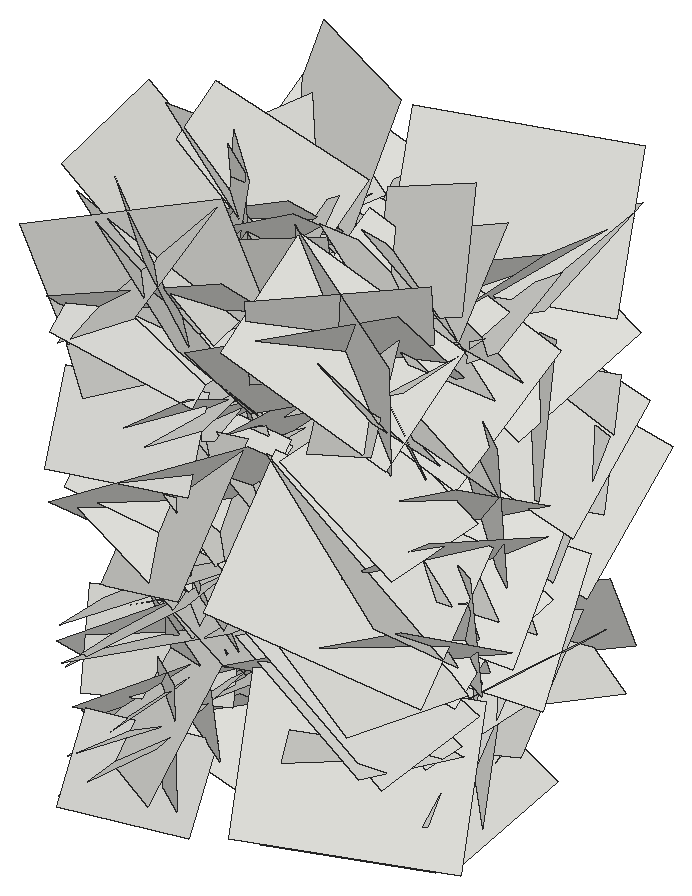
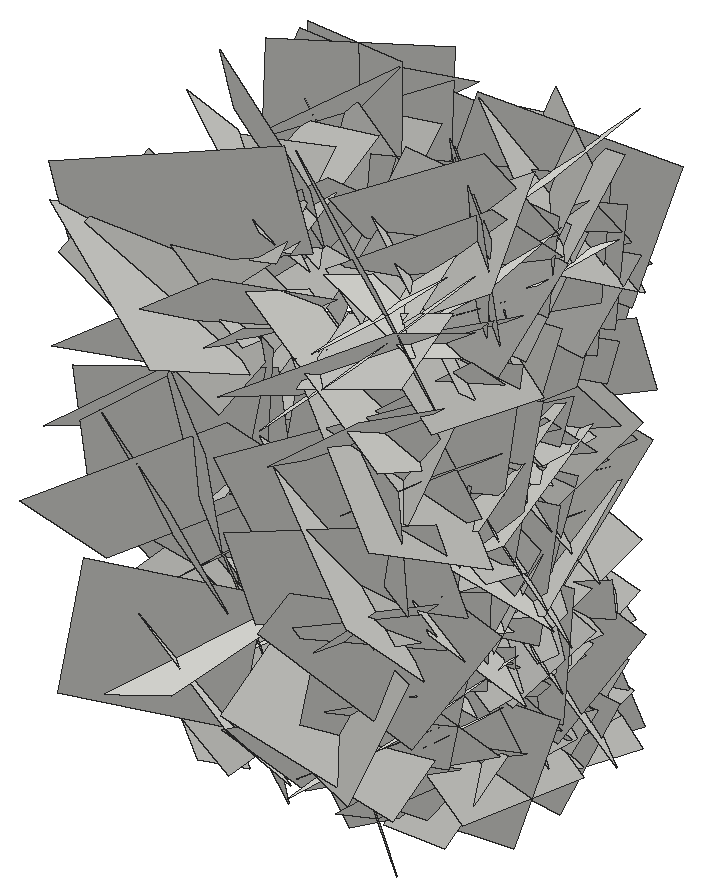
# SketchUp Ruby script. Lengths in inches.
U = 1.inch
M = Sketchup.active_model
def pt(a) = Geom::Point3d.new(a.map { |v| v * U })
def face(e, loops, mat)
  f = e.add_face(loops[0].map { |a| pt(a) })
  loops[1..].each { |l| e.add_face(l.map { |a| pt(a) }).erase! }
  f.material = f.back_material = mat if mat
  f
end
# faces: each face lists its corners as indices into pts; further lists are holes
def faces(e, pts, list, mat = nil) = list.each { |f| face(e, (f[0].is_a?(Array) ? f : [f]).map { |l| l.map { |i| pts[i] } }, mat) }
# xy, xz, yz: faces in a plane at the given z, y or x. An outline is a flat list of corners, or four numbers for a rectangle; further outlines are holes
def ring(l) = l.size == 4 ? [[l[0], l[1]], [l[2], l[1]], [l[2], l[3]], [l[0], l[3]]] : l.each_slice(2).to_a
def flat(e, list, mat, &to3) = list.each { |f| face(e, (f[0].is_a?(Array) ? f : [f]).map { |l| ring(l).map { |u, v| to3.(u, v) } }, mat) }
def xy(e, z, list, mat = nil) = flat(e, list, mat) { |x, y| [x, y, z] }
def xz(e, y, list, mat = nil) = flat(e, list, mat) { |x, z| [x, y, z] }
def yz(e, x, list, mat = nil) = flat(e, list, mat) { |y, z| [x, y, z] }
def lines(e, pts, list) = list.each { |a, b| e.add_line(pt(pts[a]), pt(pts[b])) }
# prism: a flat outline (further loops are holes) pulled along v
def prism(e, loops, v, mat = nil)
  f = face(e, loops, mat); d = Geom::Vector3d.new(v.map { |x| x * U })
  f.pushpull(f.normal.samedirection?(d) ? d.length : -d.length)
end
def box(e, o, s, mat = nil) = prism(e, [[o, [o[0] + s[0], o[1], o[2]], [o[0] + s[0], o[1] + s[1], o[2]], [o[0], o[1] + s[1], o[2]]]], [0, 0, s[2]], mat)
def at(x, y, z, deg = 0) = Geom::Transformation.translation(pt([x, y, z])) * Geom::Transformation.rotation(ORIGIN, Z_AXIS, deg.degrees)
def axes(o, x, y, z) = Geom::Transformation.new([*x, 0, *y, 0, *z, 0, *pt(o).to_a, 1])
def part(name) = M.definitions.add(name)
# library, detail: a bought-in or finely detailed component or shape, given as its bounding box
def library(name, o, s) = part(name).tap { |d| box(d.entities, o, s) }
def detail(e, o, s) = box(e.add_group.entities, o, s)
def put(e, d, t, mat = nil) = e.add_instance(d, t).tap { |i| i.material = mat if mat }
def group(e, t, mat = nil) = e.add_group.tap { |g| g.transformation = t; g.material = mat if mat }.entities
root = M.entities
c1 = part("Component\#6")
p = [[0.01,0,0],[0,3.24,4.54],[4.32,3.24,4.54],[4.33,0,0]]
faces(c1.entities,p,[[0,1,2,3]])
put(root,c1,axes([24.34,188.38,23.95],[-0.14683,-0.05211,-1.06804],[-0.1506,-1.06652,0.07046],[1.12342,-0.14978,-0.13015]))
put(root,c1,axes([28.31,187.95,18.35],[0.24952,-0.85217,0.60628],[0.01294,0.62364,0.87183],[-1.1085,-0.18454,0.14665]))
put(root,c1,axes([28.31,184.68,7.1],[0.07537,-0.21143,-0.85755],[0.01444,-0.85996,0.21315],[-0.93612,-0.03029,-0.06575]))
put(root,c1,axes([24.34,184.16,21.8125],[-0.07155,0.99261,-0.10082],[-0.11355,-0.10768,-0.9884],[1.05147,0.05592,-0.1136]))
put(root,c1,axes([24.34,192.04,5.47],[-0.24252,-0.79203,0.72828],[-0.0092,0.7459,0.80846],[1.14049,-0.1624,0.16139]))
put(root,c1,axes([24.34,189.65,5.54],[0.06955,0.77959,0.08211],[0.00823,0.08175,-0.78235],[0.8309,-0.06607,0.00087]))
put(root,c1,axes([24.34,189.86,21.06],[-0.09411,0.75469,-0.30292],[0.23058,-0.27158,-0.74036],[0.83059,0.16091,0.17121]))
put(root,c1,axes([24.34,184.33,2.33],[-0.23495,-0.78095,0.69461],[0.033,0.70481,0.80235],[1.10738,-0.18669,0.12346]))
put(root,c1,axes([28.31,182.875,15.8],[0.04284,-0.30855,-0.78276],[0.017,-0.78324,0.30957],[-0.8917,-0.02976,-0.0317]))
put(root,c1,axes([28.31,183.91,5.17],[0.1157,0.58195,-0.7538],[0.08085,-0.76164,-0.57696],[-1.0062,0.00571,-0.13304]))
put(root,c1,axes([28.31,180.19,4.07],[-0.08532,0.68038,-0.07405],[-0.04058,-0.07892,-0.68351],[-0.72433,-0.07573,0.04702]))
put(root,c1,axes([28.31,182.98,9.92],[-0.09782,-0.62966,-0.10425],[-0.08997,-0.09229,0.63256],[-0.67052,0.10424,-0.06967]))
put(root,c1,axes([28.31,190.84,12.42],[-0.00848,-0.77925,-0.15089],[0.03038,-0.15108,0.77873],[-0.8408,0.0024,0.02966]))
put(root,c1,axes([28.31,191.35,2.27],[0.06694,-0.86655,-0.10749],[0.04783,-0.10439,0.86806],[-0.92435,-0.06816,0.03713]))
put(root,c1,axes([28.31,191.46,9.82],[0.08538,-0.06629,-0.92063],[0.09555,-0.91915,0.07407],[-0.97372,-0.09601,-0.07345]))
put(root,c1,axes([28.31,193.37,9.31],[0.05697,-0.46717,-0.61186],[-0.09106,-0.61316,0.46062],[-0.81091,0.03603,-0.09471]))
put(root,c1,axes([28.31,183.28,17.73],[0.09647,-0.26045,0.74001],[-0.11879,0.73302,0.27177],[-0.82305,-0.13632,0.04751]))
put(root,c1,axes([28.31,185.14,8.49],[-0.08576,-0.66072,-0.04627],[-0.0456,-0.04128,0.66459],[-0.70059,0.08356,-0.03759]))
put(root,c1,axes([28.31,192.03,8.33],[0.03388,0.22508,-0.86549],[0.13142,-0.8588,-0.21876],[-0.93879,-0.1121,-0.06186]))
put(root,c1,axes([24.34,192.08,20.31],[0.05296,-0.67773,-0.30339],[0.1724,-0.2867,0.66724],[0.76797,0.11109,-0.12886]))
put(root,c1,axes([24.34,184.53,11.29],[-0.10396,-0.95246,0.37472],[-0.04499,0.37989,0.95451],[1.084,-0.07558,0.07555]))
put(root,c1,axes([28.31,183.19,13.8],[0.02762,0.65605,0.3231],[-0.06014,0.32414,-0.6536],[-0.77284,-0.00178,0.06241]))
put(root,c1,axes([28.31,185.94,13.1875],[0.12339,0.16979,-0.82402],[-0.01755,-0.83125,-0.17361],[-0.89164,0.03986,-0.11061]))
put(root,c1,axes([28.31,185.26,12.26],[0.159,0.84642,0.10737],[-0.04855,0.11685,-0.85715],[-0.9031,0.14274,0.06498]))
put(root,c1,axes([24.34,181.6,11.88],[0.05183,0.72565,0.67247],[-0.15864,0.67097,-0.71314],[1.03662,0.0664,-0.14276]))
put(root,c1,axes([28.31,192.38,19.24],[-0.04943,-0.7355,0.057],[0.07325,0.05251,0.73407],[-0.77853,0.05163,0.06545]))
put(root,c1,axes([24.34,185.13,2.21],[0.09174,0.69928,0.36],[0.10121,0.35015,-0.7031],[0.82753,-0.12035,0.04608]))
put(root,c1,axes([24.34,185.25,15.47],[0.04372,0.77316,0.71524],[-0.20224,0.70943,-0.75587],[1.09798,0.09988,-0.16771]))
put(root,c1,axes([24.34,183.61,1.59],[0.06331,-0.78644,0.46242],[-0.03597,0.46118,0.7887],[0.96639,0.06869,-0.00094]))
put(root,c1,axes([24.34,186.63,-0.64],[-0.14781,-0.37723,1.01914],[-0.01271,1.02797,0.37886],[1.15185,-0.03706,0.13496]))
put(root,c1,axes([24.34,183.46,7.83],[-0.1867,0.36795,-0.96583],[0.13041,-0.96532,-0.39019],[1.08777,0.17888,-0.11899]))
put(root,c1,axes([28.31,192.83,7.86],[-0.1126,-0.65912,-0.17655],[0.1088,-0.19208,0.65534],[-0.71507,0.07456,0.12751]))
put(root,c1,axes([28.31,183.375,2.21],[-0.01982,-0.33114,-0.74136],[0.16849,-0.7287,0.32148],[-0.84401,-0.13769,0.08159]))
put(root,c1,axes([24.34,187.85,22.99],[0.09057,-0.06637,-0.91857],[-0.07612,-0.92019,0.05981],[0.97325,-0.06579,0.09016]))
put(root,c1,axes([24.34,187.17,12.95],[-0.05814,-0.16279,1.09674],[-0.14666,1.09051,0.15494],[1.1661,0.12904,0.07417]))
put(root,c1,axes([24.34,185.08,2.16],[0.06404,-1.02262,-0.11109],[-0.17979,-0.11966,1.00929],[1.07543,0.04089,0.17535]))
put(root,c1,axes([24.34,180.14,11.99],[-0.0212,0.75168,0.8023],[-0.17372,0.79143,-0.74558],[1.15236,0.13314,-0.09764]))
put(root,c1,axes([28.31,186.92,8.78],[0.10246,-0.30095,0.75916],[0.04625,0.76527,0.29782],[-0.86439,0.00528,0.10592]))
put(root,c1,axes([24.34,191,16.96],[-0.17643,-1.14926,-0.11809],[-0.05518,-0.11173,1.16072],[1.22339,-0.17078,0.03532]))
put(root,c1,axes([24.34,189.57,16.9],[0.06471,0.53395,-0.71324],[0.01751,-0.71546,-0.53421],[0.94426,-0.02333,0.05878]))
put(root,c1,axes([28.31,184.43,15.42],[0.12844,-0.04329,0.74472],[-0.08874,0.74892,0.05716],[-0.78574,-0.09166,0.11528]))
put(root,c1,axes([24.34,179.97,24.47],[-0.23304,1.36821,0.06434],[-0.25904,0.02493,-1.36533],[1.42861,0.2277,-0.23708]))
put(root,c1,axes([24.34,190.33,17.67],[0.17424,0.82504,0.17436],[-0.04616,0.18571,-0.83769],[0.89267,-0.15144,-0.07735]))
put(root,c1,axes([24.34,186.72,4.72],[-0.08241,-0.91883,0.29273],[0.13826,0.28096,0.91654],[1.0128,-0.11312,-0.1013]))
put(root,c1,axes([24.34,185.64,19.96],[-0.2349,1.07139,0.39402],[0.08081,0.41437,-1.08385],[1.20734,0.18072,0.1492]))
put(root,c1,axes([28.31,184.54,3.47],[0.05739,0.5962,-0.42459],[0.0201,-0.42675,-0.59681],[-0.77559,0.03305,-0.04688]))
put(root,c1,axes([28.31,189.45,1.42],[-0.1039,0.30381,0.53974],[0.07033,0.54846,-0.29667],[-0.65275,0.01074,-0.11787]))
put(root,c1,axes([24.34,186.9375,3.03],[0.11563,0.62873,-0.58509],[0.05581,-0.59358,-0.62803],[0.90867,-0.04354,0.11303]))
put(root,c1,axes([24.34,184.51,1.15],[-0.01173,-1.06899,-0.22188],[-0.10644,-0.21996,1.06472],[1.15237,-0.0312,0.09608]))
put(root,c1,axes([28.31,183.83,7.3125],[0.02805,0.62389,-0.09529],[-0.05665,-0.09282,-0.62253],[-0.66659,0.03414,0.0489]))
put(root,c1,axes([28.31,183.1,18.89],[0.1435,0.17311,-0.85276],[0.14536,-0.85648,-0.1521],[-0.91084,-0.10941,-0.15862]))
put(root,c1,axes([24.34,187.61,11.62],[-0.28203,-0.58282,-1.12773],[0.01249,-1.15332,0.59327],[1.34554,-0.11146,-0.24188]))
put(root,c1,axes([24.34,184.19,13.53],[0.08078,-0.49886,0.79857],[0.01528,0.8017,0.49945],[0.99796,0.02811,-0.07229]))
put(root,c1,axes([24.34,181.29,16.68],[0.08133,-0.245,0.96212],[-0.05676,0.96256,0.24939],[1.05086,0.07095,-0.06099]))
put(root,c1,axes([28.31,186.0625,6.1],[0.08854,0.52684,0.45627],[-0.00383,0.45985,-0.53032],[-0.73876,0.06076,0.05744]))
put(root,c1,axes([28.31,187.98,11.49],[0.12716,0.81746,0.20835],[0.15,0.18797,-0.81896],[-0.88154,0.1499,-0.10929]))
put(root,c1,axes([24.34,194.3,13.93],[-0.22437,-1.23478,-0.60854],[-0.19245,-0.58527,1.25072],[1.44644,-0.26941,0.07201]))
put(root,c1,axes([24.34,184.41,20.14],[-0.03821,-1.03167,-0.60174],[-0.15497,-0.59368,1.0266],[1.25647,-0.1046,0.10832]))
put(root,c1,axes([28.31,186.3,8.38],[-0.07617,0.47932,0.41871],[0.13681,0.42359,-0.46276],[-0.66062,0.03245,-0.14411]))
put(root,c1,axes([24.34,184.31,4.6],[0.1576,-0.1516,-1.0147],[-0.15202,-1.0183,0.13112],[1.07684,-0.12157,0.16702]))
put(root,c1,axes([24.34,179.32,18.3],[0.15069,0.54422,0.74866],[-0.00735,0.75804,-0.54972],[0.98107,-0.07791,-0.11911]))
put(root,c1,axes([28.31,188.8,6.44],[0.14743,-0.18272,-0.74199],[0.06403,-0.74919,0.19581],[-0.80747,-0.09277,-0.11994]))
put(root,c1,axes([24.34,185.52,6.2],[-0.2751,-0.65276,-1.16933],[-0.03559,-1.18754,0.67037],[1.41909,-0.15632,-0.20987]))
put(root,c1,axes([24.34,181.08,20.02],[-0.00536,1.00575,0.03656],[0.10796,0.03689,-1.00058],[1.06133,0.00133,0.10197]))
put(root,c1,axes([24.34,184.05,20.67],[0.10102,0.73684,0.6989],[-0.04073,0.70408,-0.73707],[1.07574,-0.04254,-0.09354]))
put(root,c1,axes([24.34,191.125,9.45],[-0.23474,-0.88576,-0.93612],[0.00151,-0.95001,0.89856],[1.36608,-0.15116,-0.16185]))
put(root,c1,axes([24.34,185.11,13.22],[0.08906,-0.95701,-0.12674],[0.0585,-0.12225,0.95969],[1.02162,0.09043,-0.0439]))
put(root,c1,axes([24.34,180.4,17.125],[-0.23878,-0.31981,1.17522],[0.15258,1.17979,0.34864],[1.28199,-0.19998,0.17739]))
put(root,c1,axes([24.34,187.48,17.59],[-0.04794,-0.78864,0.66349],[0.19289,0.64758,0.78214],[1.07529,-0.15133,-0.11072]))
put(root,c1,axes([24.34,187.26,9.21],[0.06299,-0.71122,-0.64775],[0.16214,-0.63375,0.70987],[1.00673,0.14657,-0.0738]))
put(root,c1,axes([28.31,191.11,1.26],[0.04561,-0.57908,-0.31344],[0.1156,-0.3035,0.57569],[-0.68833,-0.08935,0.07592]))
put(root,c1,axes([24.34,186.13,19.34],[0.13168,0.96657,0.23982],[0.01085,0.24043,-0.97432],[1.05558,-0.12304,-0.0199]))
put(root,c1,axes([24.34,188.68,19.83],[-0.08458,1.11358,0.50301],[-0.01593,0.50315,-1.11627],[1.29513,0.07891,0.01912]))
put(root,c1,axes([24.34,185.36,5.79],[0.02078,-1.22604,-0.15411],[-0.11589,-0.15525,1.22117],[1.3047,0.00574,0.11093]))
put(root,c1,axes([24.34,186.43,6.6],[-0.00451,1.27416,-0.10814],[-0.14001,-0.108,-1.26731],[1.34821,-0.00695,-0.13197]))
put(root,c1,axes([28.31,190.35,18.26],[0.16101,-0.65287,0.16772],[0.08445,0.18811,0.66008],[-0.7095,-0.12576,0.11663]))
put(root,c1,axes([24.34,187.9375,5.11],[0.04973,-1.23753,-0.07043],[-0.13139,-0.07481,1.23194],[1.30732,0.03956,0.12649]))
put(root,c1,axes([24.34,189.08,9.2],[-0.13088,0.55221,1.09741],[0.12619,1.10312,-0.54169],[1.29609,-0.05164,0.16356]))
put(root,c1,axes([24.34,182.44,13.63],[-0.1579,1.28482,-0.45217],[-0.02165,-0.45692,-1.2916],[1.44363,0.13368,-0.06883]))
put(root,c1,axes([24.34,182.53,23.48],[0.24403,0.37129,-0.99391],[-0.1038,-1.00526,-0.39821],[1.11985,-0.17408,0.17968]))
put(root,c1,axes([24.34,192.17,8.01],[0.17438,0.53527,-0.89237],[0.02164,-0.90494,-0.53904],[1.10282,-0.06688,0.15168]))
put(root,c1,axes([24.34,188.23,7.57],[0.0913,-1.12353,0.75234],[-0.27462,0.72618,1.11413],[1.40673,0.21468,0.16867]))
put(root,c1,axes([24.34,194.04,23.84],[-0.15699,-0.54259,-1.24113],[0.03696,-1.24964,0.54215],[1.43535,-0.02717,-0.14971]))
put(root,c1,axes([24.34,189.36,1.43],[-0.09807,-1.35815,-0.14277],[-0.05055,-0.1398,1.36078],[1.44669,-0.09695,0.03787]))
put(root,c1,axes([24.34,188.7,21.97],[0.14471,1.28216,-0.28655],[-0.25359,-0.25902,-1.27293],[1.36933,-0.18346,-0.20546]))
put(root,c1,axes([24.34,190.12,11.53],[-0.21117,-0.99907,-0.90649],[0.1512,-0.92678,0.99009],[1.42194,-0.04983,-0.2399]))
put(root,c1,axes([24.34,183.02,16.38],[-0.02893,-0.8566,0.75588],[0.26219,0.73373,0.84043],[1.18223,-0.18368,-0.16789]))
put(root,c1,axes([24.34,185.31,6.45],[-0.03902,-0.20515,1.15818],[0.22164,1.13915,0.20842],[1.22693,-0.21231,-0.00082]))
put(root,c1,axes([24.34,180.93,10.86],[-0.17521,1.15715,-0.62152],[0.20897,-0.59747,-1.1648],[1.37654,0.23798,0.09772]))
put(root,c1,axes([24.34,184.5,10.44],[0.20009,0.552,-0.98447],[-0.02572,-0.99592,-0.56307],[1.1961,-0.11375,0.15258]))
put(root,c1,axes([24.34,185.25,0.97],[0.15144,0.45294,1.0525],[0.02813,1.05906,-0.45936],[1.21425,-0.08102,-0.12063]))
put(root,c1,axes([24.34,182.38,2.76],[0.16715,0.82367,0.72398],[0.09449,0.71938,-0.83785],[1.15857,-0.1775,-0.03612]))
put(root,c1,axes([24.34,186.66,10.07],[-0.09303,-0.2424,1.37134],[-0.00293,1.37409,0.24271],[1.47615,-0.01254,0.08691]))
put(root,c1,axes([24.34,192.77,15.58],[0.03721,-0.16955,-1.17702],[0.1418,-1.1695,0.17246],[1.25252,0.13744,0.01545]))
put(root,c1,axes([24.34,185.87,11.99],[0.00632,-0.88407,-1.06115],[-0.10628,-1.05864,0.88141],[1.46017,-0.07323,0.06874]))
put(root,c1,axes([24.34,186.02,17.55],[0.12484,-0.91824,0.67786],[0.09261,0.68671,0.91505],[1.20627,0.04231,-0.14041]))
put(root,c1,axes([24.34,195.54,11.625],[0.04246,-1.00606,-0.92627],[-0.11693,-0.92602,1.00103],[1.44486,-0.04538,0.10823]))
put(root,c1,axes([24.34,183.88,15.08],[-0.0404,1.11797,-0.62329],[0.16276,-0.61507,-1.11262],[1.34698,0.10785,0.11575]))
put(root,c1,axes([24.34,184.23,21.55],[0.30098,0.54789,0.85036],[0.10123,0.86476,-0.58905],[1.06749,-0.23649,-0.1839]))
put(root,c1,axes([24.34,184,8.18],[-0.02134,-1.06466,0.81449],[0.04088,0.81378,1.06469],[1.42032,-0.03942,-0.01841]))
put(root,c1,axes([24.34,188.34,12.62],[0.20954,0.481,1.15591],[-0.07101,1.17261,-0.47649],[1.32521,-0.01322,-0.2083]))
put(root,c1,axes([24.34,186.39,13.5625],[0.22643,-0.80881,0.81079],[0.0736,0.83241,0.81208],[1.21171,0.10058,-0.20084]))
put(root,c1,axes([24.34,184.34,4.6],[0.11485,-1.15497,0.26483],[0.19184,0.27894,1.14248],[1.2413,0.06375,-0.20107]))
put(root,c1,axes([24.34,193.03,3.2],[0.23388,-1.096,0.27231],[0.13541,0.2999,1.10354],[1.1894,0.18138,-0.17918]))
put(root,c1,axes([24.34,189.55,17.94],[0.16397,-1.09761,-0.83604],[-0.11999,-0.84854,1.09307],[1.45761,0.05363,0.18403]))
put(root,c1,axes([24.34,187.39,3.1875],[0.10139,0.89849,0.89189],[0.1671,0.87902,-0.90243],[1.33152,-0.17873,0.04534]))
put(root,c1,axes([24.34,180.76,23.09],[0.06995,0.91309,-0.96842],[0.10566,-0.97028,-0.90805],[1.4069,0.02747,0.11634]))
put(root,c1,axes([24.34,183.54,2.14],[0.03864,0.84179,0.92004],[0.33491,0.88417,-0.82148],[1.27872,-0.257,0.18735]))
put(root,c1,axes([24.34,184.58,6.82],[0.16596,-1.29847,0.14138],[0.0614,0.14916,1.30572],[1.38315,0.14917,-0.07492]))
put(root,c1,axes([24.34,193.85,16.74],[0.30124,-1.14539,-0.57535],[-0.00001,-0.58933,1.17321],[1.35869,0.25394,0.12757]))
put(root,c1,axes([24.34,189.11,8.53],[0.25892,-1.11224,-0.53402],[0.14932,-0.51568,1.13849],[1.29927,0.28091,-0.02442]))
put(root,c1,axes([24.34,182.27,16.13],[0.23771,-0.47409,1.27281],[0.00404,1.29026,0.47991],[1.43973,0.07465,-0.2115]))
put(root,c1,axes([38.11,182.27,16.13],[-0.23771,-0.47409,1.27281],[-0.00404,1.29026,0.47991],[-1.43973,0.07465,-0.2115]))
put(root,c1,axes([38.11,189.11,8.53],[-0.25892,-1.11224,-0.53402],[-0.14932,-0.51568,1.13849],[-1.29927,0.28091,-0.02442]))
put(root,c1,axes([38.11,193.85,16.74],[-0.30124,-1.14539,-0.57535],[0.00001,-0.58933,1.17321],[-1.35869,0.25394,0.12757]))
put(root,c1,axes([38.11,184.58,6.82],[-0.16596,-1.29847,0.14138],[-0.0614,0.14916,1.30572],[-1.38315,0.14917,-0.07492]))
put(root,c1,axes([38.11,183.54,2.14],[-0.03864,0.84179,0.92004],[-0.33491,0.88417,-0.82148],[-1.27872,-0.257,0.18735]))
put(root,c1,axes([38.11,180.76,23.09],[-0.06995,0.91309,-0.96842],[-0.10566,-0.97028,-0.90805],[-1.4069,0.02747,0.11634]))
put(root,c1,axes([38.11,187.39,3.1875],[-0.10139,0.89849,0.89189],[-0.1671,0.87902,-0.90243],[-1.33152,-0.17873,0.04534]))
put(root,c1,axes([38.11,189.55,17.94],[-0.16397,-1.09761,-0.83604],[0.11999,-0.84854,1.09307],[-1.45761,0.05363,0.18403]))
put(root,c1,axes([38.11,193.03,3.2],[-0.23388,-1.096,0.27231],[-0.13541,0.2999,1.10354],[-1.1894,0.18138,-0.17918]))
put(root,c1,axes([38.11,184.34,4.6],[-0.11485,-1.15497,0.26483],[-0.19184,0.27894,1.14248],[-1.2413,0.06375,-0.20107]))
put(root,c1,axes([38.11,186.39,13.5625],[-0.22643,-0.80881,0.81079],[-0.0736,0.83241,0.81208],[-1.21171,0.10058,-0.20084]))
put(root,c1,axes([38.11,188.34,12.62],[-0.20954,0.481,1.15591],[0.07101,1.17261,-0.47649],[-1.32521,-0.01322,-0.2083]))
put(root,c1,axes([38.11,184,8.18],[0.02134,-1.06466,0.81449],[-0.04088,0.81378,1.06469],[-1.42032,-0.03942,-0.01841]))
put(root,c1,axes([38.11,184.23,21.55],[-0.30098,0.54789,0.85036],[-0.10123,0.86476,-0.58905],[-1.06749,-0.23649,-0.1839]))
put(root,c1,axes([38.11,183.88,15.08],[0.0404,1.11797,-0.62329],[-0.16276,-0.61507,-1.11262],[-1.34698,0.10785,0.11575]))
put(root,c1,axes([38.11,195.54,11.625],[-0.04246,-1.00606,-0.92627],[0.11693,-0.92602,1.00103],[-1.44486,-0.04538,0.10823]))
put(root,c1,axes([38.11,186.02,17.55],[-0.12484,-0.91824,0.67786],[-0.09261,0.68671,0.91505],[-1.20627,0.04231,-0.14041]))
put(root,c1,axes([38.11,185.87,11.99],[-0.00632,-0.88407,-1.06115],[0.10628,-1.05864,0.88141],[-1.46017,-0.07323,0.06874]))
put(root,c1,axes([38.11,192.77,15.58],[-0.03721,-0.16955,-1.17702],[-0.1418,-1.1695,0.17246],[-1.25252,0.13744,0.01545]))
put(root,c1,axes([38.11,186.66,10.07],[0.09303,-0.2424,1.37134],[0.00293,1.37409,0.24271],[-1.47615,-0.01254,0.08691]))
put(root,c1,axes([38.11,182.38,2.76],[-0.16715,0.82367,0.72398],[-0.09449,0.71938,-0.83785],[-1.15857,-0.1775,-0.03612]))
put(root,c1,axes([38.11,185.25,0.97],[-0.15144,0.45294,1.0525],[-0.02813,1.05906,-0.45936],[-1.21425,-0.08102,-0.12063]))
put(root,c1,axes([38.11,184.5,10.44],[-0.20009,0.552,-0.98447],[0.02572,-0.99592,-0.56307],[-1.1961,-0.11375,0.15258]))
put(root,c1,axes([38.11,180.93,10.86],[0.17521,1.15715,-0.62152],[-0.20897,-0.59747,-1.1648],[-1.37654,0.23798,0.09772]))
put(root,c1,axes([38.11,185.31,6.45],[0.03902,-0.20515,1.15818],[-0.22164,1.13915,0.20842],[-1.22693,-0.21231,-0.00082]))
put(root,c1,axes([38.11,183.02,16.38],[0.02893,-0.8566,0.75588],[-0.26219,0.73373,0.84043],[-1.18223,-0.18368,-0.16789]))
put(root,c1,axes([38.11,190.12,11.53],[0.21117,-0.99907,-0.90649],[-0.1512,-0.92678,0.99009],[-1.42194,-0.04983,-0.2399]))
put(root,c1,axes([38.11,188.7,21.97],[-0.14471,1.28216,-0.28655],[0.25359,-0.25902,-1.27293],[-1.36933,-0.18346,-0.20546]))
put(root,c1,axes([38.11,189.36,1.43],[0.09807,-1.35815,-0.14277],[0.05055,-0.1398,1.36078],[-1.44669,-0.09695,0.03787]))
put(root,c1,axes([38.11,194.04,23.84],[0.15699,-0.54259,-1.24113],[-0.03696,-1.24964,0.54215],[-1.43535,-0.02717,-0.14971]))
put(root,c1,axes([38.11,188.23,7.57],[-0.0913,-1.12353,0.75234],[0.27462,0.72618,1.11413],[-1.40673,0.21468,0.16867]))
put(root,c1,axes([38.11,192.17,8.01],[-0.17438,0.53527,-0.89237],[-0.02164,-0.90494,-0.53904],[-1.10282,-0.06688,0.15168]))
put(root,c1,axes([38.11,182.53,23.48],[-0.24403,0.37129,-0.99391],[0.1038,-1.00526,-0.39821],[-1.11985,-0.17408,0.17968]))
put(root,c1,axes([38.11,182.44,13.63],[0.1579,1.28482,-0.45217],[0.02165,-0.45692,-1.2916],[-1.44363,0.13368,-0.06883]))
put(root,c1,axes([38.11,189.08,9.2],[0.13088,0.55221,1.09741],[-0.12619,1.10312,-0.54169],[-1.29609,-0.05164,0.16356]))
put(root,c1,axes([38.11,187.9375,5.11],[-0.04973,-1.23753,-0.07043],[0.13139,-0.07481,1.23194],[-1.30732,0.03956,0.12649]))
put(root,c1,axes([34.14,190.35,18.26],[-0.16101,-0.65287,0.16772],[-0.08445,0.18811,0.66008],[0.7095,-0.12576,0.11663]))
put(root,c1,axes([38.11,186.43,6.6],[0.00451,1.27416,-0.10814],[0.14001,-0.108,-1.26731],[-1.34821,-0.00695,-0.13197]))
put(root,c1,axes([38.11,185.36,5.79],[-0.02078,-1.22604,-0.15411],[0.11589,-0.15525,1.22117],[-1.3047,0.00574,0.11093]))
put(root,c1,axes([38.11,188.68,19.83],[0.08458,1.11358,0.50301],[0.01593,0.50315,-1.11627],[-1.29513,0.07891,0.01912]))
put(root,c1,axes([38.11,186.13,19.34],[-0.13168,0.96657,0.23982],[-0.01085,0.24043,-0.97432],[-1.05558,-0.12304,-0.0199]))
put(root,c1,axes([34.14,191.11,1.26],[-0.04561,-0.57908,-0.31344],[-0.1156,-0.3035,0.57569],[0.68833,-0.08935,0.07592]))
put(root,c1,axes([38.11,187.26,9.21],[-0.06299,-0.71122,-0.64775],[-0.16214,-0.63375,0.70987],[-1.00673,0.14657,-0.0738]))
put(root,c1,axes([38.11,187.48,17.59],[0.04794,-0.78864,0.66349],[-0.19289,0.64758,0.78214],[-1.07529,-0.15133,-0.11072]))
put(root,c1,axes([38.11,180.4,17.125],[0.23878,-0.31981,1.17522],[-0.15258,1.17979,0.34864],[-1.28199,-0.19998,0.17739]))
put(root,c1,axes([38.11,185.11,13.22],[-0.08906,-0.95701,-0.12674],[-0.0585,-0.12225,0.95969],[-1.02162,0.09043,-0.0439]))
put(root,c1,axes([38.11,191.125,9.45],[0.23474,-0.88576,-0.93612],[-0.00151,-0.95001,0.89856],[-1.36608,-0.15116,-0.16185]))
put(root,c1,axes([38.11,184.05,20.67],[-0.10102,0.73684,0.6989],[0.04073,0.70408,-0.73707],[-1.07574,-0.04254,-0.09354]))
put(root,c1,axes([38.11,181.08,20.02],[0.00536,1.00575,0.03656],[-0.10796,0.03689,-1.00058],[-1.06133,0.00133,0.10197]))
put(root,c1,axes([38.11,185.52,6.2],[0.2751,-0.65276,-1.16933],[0.03559,-1.18754,0.67037],[-1.41909,-0.15632,-0.20987]))
put(root,c1,axes([34.14,188.8,6.44],[-0.14743,-0.18272,-0.74199],[-0.06403,-0.74919,0.19581],[0.80747,-0.09277,-0.11994]))
put(root,c1,axes([38.11,179.32,18.3],[-0.15069,0.54422,0.74866],[0.00735,0.75804,-0.54972],[-0.98107,-0.07791,-0.11911]))
put(root,c1,axes([38.11,184.31,4.6],[-0.1576,-0.1516,-1.0147],[0.15202,-1.0183,0.13112],[-1.07684,-0.12157,0.16702]))
put(root,c1,axes([34.14,186.3,8.38],[0.07617,0.47932,0.41871],[-0.13681,0.42359,-0.46276],[0.66062,0.03245,-0.14411]))
put(root,c1,axes([38.11,184.41,20.14],[0.03821,-1.03167,-0.60174],[0.15497,-0.59368,1.0266],[-1.25647,-0.1046,0.10832]))
put(root,c1,axes([38.11,194.3,13.93],[0.22437,-1.23478,-0.60854],[0.19245,-0.58527,1.25072],[-1.44644,-0.26941,0.07201]))
